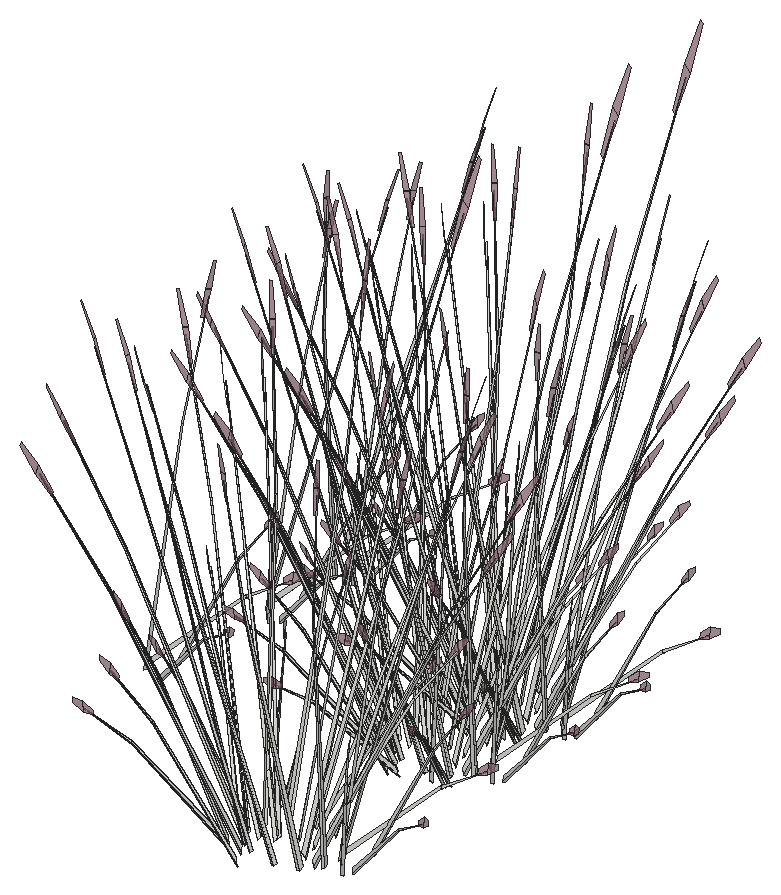
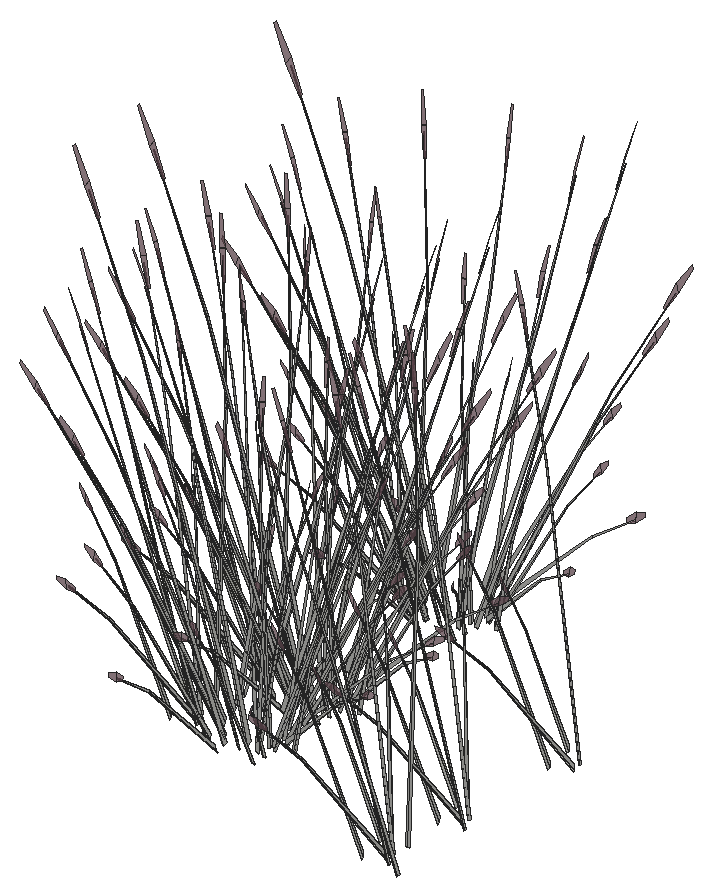
# SketchUp Ruby script. Lengths in inches.
U = 1.inch
M = Sketchup.active_model
def pt(a) = Geom::Point3d.new(a.map { |v| v * U })
def face(e, loops, mat)
  f = e.add_face(loops[0].map { |a| pt(a) })
  loops[1..].each { |l| e.add_face(l.map { |a| pt(a) }).erase! }
  f.material = f.back_material = mat if mat
  f
end
# faces: each face lists its corners as indices into pts; further lists are holes
def faces(e, pts, list, mat = nil) = list.each { |f| face(e, (f[0].is_a?(Array) ? f : [f]).map { |l| l.map { |i| pts[i] } }, mat) }
# xy, xz, yz: faces in a plane at the given z, y or x. An outline is a flat list of corners, or four numbers for a rectangle; further outlines are holes
def ring(l) = l.size == 4 ? [[l[0], l[1]], [l[2], l[1]], [l[2], l[3]], [l[0], l[3]]] : l.each_slice(2).to_a
def flat(e, list, mat, &to3) = list.each { |f| face(e, (f[0].is_a?(Array) ? f : [f]).map { |l| ring(l).map { |u, v| to3.(u, v) } }, mat) }
def xy(e, z, list, mat = nil) = flat(e, list, mat) { |x, y| [x, y, z] }
def xz(e, y, list, mat = nil) = flat(e, list, mat) { |x, z| [x, y, z] }
def yz(e, x, list, mat = nil) = flat(e, list, mat) { |y, z| [x, y, z] }
def lines(e, pts, list) = list.each { |a, b| e.add_line(pt(pts[a]), pt(pts[b])) }
# prism: a flat outline (further loops are holes) pulled along v
def prism(e, loops, v, mat = nil)
  f = face(e, loops, mat); d = Geom::Vector3d.new(v.map { |x| x * U })
  f.pushpull(f.normal.samedirection?(d) ? d.length : -d.length)
end
def box(e, o, s, mat = nil) = prism(e, [[o, [o[0] + s[0], o[1], o[2]], [o[0] + s[0], o[1] + s[1], o[2]], [o[0], o[1] + s[1], o[2]]]], [0, 0, s[2]], mat)
def at(x, y, z, deg = 0) = Geom::Transformation.translation(pt([x, y, z])) * Geom::Transformation.rotation(ORIGIN, Z_AXIS, deg.degrees)
def axes(o, x, y, z) = Geom::Transformation.new([*x, 0, *y, 0, *z, 0, *pt(o).to_a, 1])
def part(name) = M.definitions.add(name)
# library, detail: a bought-in or finely detailed component or shape, given as its bounding box
def library(name, o, s) = part(name).tap { |d| box(d.entities, o, s) }
def detail(e, o, s) = box(e.add_group.entities, o, s)
def put(e, d, t, mat = nil) = e.add_instance(d, t).tap { |i| i.material = mat if mat }
def group(e, t, mat = nil) = e.add_group.tap { |g| g.transformation = t; g.material = mat if mat }.entities
root = M.entities
M.materials.add("LightPink_Translucent").color = [144, 107, 117]
M.materials["LightPink_Translucent"].alpha = 0.75
c1 = part("blade")
p = [[2.15,0.21,22],[0,0.17,0],[0.09,0.45,0],[2.18,0.31,22],[2.29,0.31,22],[0.38,0.45,0],
  [2.48,0.24,33],[2.49,0.24,33],[2.48,0.22,33]]
faces(c1.entities,p,[[0,1,2,3],[4,5,2,3],[6,3,4,7],[8,0,3,6]])
c2 = part("seeds")
p = [[0.3,-0.1,1.38],[-0.01,-0.03,1.59],[-0.01,-0.03,0.03],[0.14,-0.07,-0.07],[0.29,-0.03,3],[0.15,0.01,3.11]]
faces(c2.entities,p,[[0,1,2,3],[1,0,4,5]],"LightPink_Translucent")
c3 = part("blade with seeds")
put(c3.entities,c1,at(0,0,0))
put(c3.entities,c2,axes([2.4,0.25,30.99],[1.5799,-0.05474,1.17369],[-0.12525,1.92788,0.29478],[-0.07173,-0.02425,1.56792]))
put(root,c3,axes([679.98,333.62,514.18],[-0.32734,-0.51701,-0.10093],[0.58097,-0.25407,-0.56021],[0.24483,-0.06821,0.85122]))
put(root,c3,axes([679.89,351.33,514.18],[0.38768,-0.48872,-0.10093],[0.56143,0.28156,-0.56021],[0.19516,0.13808,0.85122]))
put(root,c3,axes([681.9,348.4,514.18],[-0.60181,-0.31483,-0.10093],[0.34671,-0.45593,-0.56021],[0.17003,-0.15849,0.85122]))
put(root,c3,axes([679.82,334.35,513.91],[0.13956,-0.00966,1.45204],[0.38281,-0.44358,-0.22964],[0.24825,0.05855,0.11645]))
put(root,c3,axes([682.43,341.93,513.91],[-0.08498,-0.00434,1.47228],[-0.35287,-0.46464,-0.13912],[0.14171,-0.15278,0.26054]))
put(root,c3,axes([680.24,344.37,514.18],[0.03484,-0.58066,-0.10093],[0.65957,0.01587,-0.56021],[0.25402,0.04034,0.85122]))
put(root,c3,axes([680.97,343.3,514.18],[-0.32734,-0.51701,-0.10093],[0.58097,-0.25407,-0.56021],[0.24483,-0.06821,0.85122]))
put(root,c3,axes([681.28,335.16,513.91],[-0.05883,-0.04999,1.47228],[0.12868,-0.53581,-0.13912],[0.23172,-0.03423,0.26054]))
put(root,c3,axes([680.81,344.02,513.91],[0.13956,-0.00966,1.45204],[0.38281,-0.44358,-0.22964],[0.24825,0.05855,0.11645]))
put(root,c3,axes([683.38,348.26,513.91],[-0.08498,-0.00434,1.47228],[-0.35287,-0.46464,-0.13912],[0.14171,-0.15278,0.26054]))
put(root,c3,axes([681.76,332.81,513.91],[0.09028,-0.08697,1.45204],[-0.11555,-0.53348,-0.22964],[0.22652,-0.10115,0.11645]))
put(root,c3,axes([681.1875,350.7,514.18],[0.03484,-0.58066,-0.10093],[0.65957,0.01587,-0.56021],[0.25402,0.04034,0.85122]))
put(root,c3,axes([681.92,349.63,514.18],[-0.32734,-0.51701,-0.10093],[0.58097,-0.25407,-0.56021],[0.24483,-0.06821,0.85122]))
put(root,c3,axes([682.27,344.83,513.91],[-0.05883,-0.04999,1.47228],[0.12868,-0.53581,-0.13912],[0.23172,-0.03423,0.26054]))
put(root,c3,axes([681.76,350.35,513.91],[0.13956,-0.00966,1.45204],[0.38281,-0.44358,-0.22964],[0.24825,0.05855,0.11645]))
put(root,c3,axes([682.75,342.49,513.91],[0.09028,-0.08697,1.45204],[-0.11555,-0.53348,-0.22964],[0.22652,-0.10115,0.11645]))
put(root,c3,axes([683.22,351.16,513.91],[-0.05883,-0.04999,1.47228],[0.12868,-0.53581,-0.13912],[0.23172,-0.03423,0.26054]))
put(root,c3,axes([683.7,348.82,513.91],[0.09028,-0.08697,1.45204],[-0.11555,-0.53348,-0.22964],[0.22652,-0.10115,0.11645]))
put(root,c3,axes([696.37,321.97,513.22],[0.26985,-0.01293,1.42242],[-0.17902,0.56047,0.11501],[-0.38456,-0.03467,0.60807]))
put(root,c3,axes([696.37,335.47,513.22],[0.26985,-0.01293,1.42242],[-0.17902,0.56047,0.11501],[-0.38456,-0.03467,0.60807]))
put(root,c3,axes([696.37,341.87,513.22],[0.26985,-0.01293,1.42242],[-0.17902,0.56047,0.11501],[-0.38456,-0.03467,0.60807]))
put(root,c3,axes([696.48,322.95,513.22],[0.22574,-0.12077,1.42242],[0.19004,0.55807,0.11501],[-0.35439,0.12613,0.60807]))
put(root,c3,axes([696.48,336.45,513.22],[0.22574,-0.12077,1.42242],[0.19004,0.55807,0.11501],[-0.35439,0.12613,0.60807]))
put(root,c3,axes([696.48,342.85,513.22],[0.22574,-0.12077,1.42242],[0.19004,0.55807,0.11501],[-0.35439,0.12613,0.60807]))
put(root,c3,axes([695.79,322.76,513.91],[-0.10624,0.07413,1.45204],[0.00904,0.54162,-0.22964],[-0.24352,0.07044,0.11645]))
put(root,c3,axes([695.79,336.26,513.91],[-0.10624,0.07413,1.45204],[0.00904,0.54162,-0.22964],[-0.24352,0.07044,0.11645]))
put(root,c3,axes([695.79,342.66,513.91],[-0.10624,0.07413,1.45204],[0.00904,0.54162,-0.22964],[-0.24352,0.07044,0.11645]))
put(root,c3,axes([696.875,321.07,513.22],[0.24166,0.09837,1.42242],[-0.50011,0.41269,0.11501],[-0.3117,-0.18617,0.60807]))
put(root,c3,axes([696.875,334.57,513.22],[0.24166,0.09837,1.42242],[-0.50011,0.41269,0.11501],[-0.3117,-0.18617,0.60807]))
put(root,c3,axes([696.875,340.97,513.22],[0.24166,0.09837,1.42242],[-0.50011,0.41269,0.11501],[-0.3117,-0.18617,0.60807]))
put(root,c3,axes([694.61,323.31,513.91],[0.08303,0.01531,1.47228],[0.25685,0.50448,-0.13912],[-0.16996,0.13241,0.26054]))
put(root,c3,axes([694.61,336.81,513.91],[0.08303,0.01531,1.47228],[0.25685,0.50448,-0.13912],[-0.16996,0.13241,0.26054]))
put(root,c3,axes([694.61,343.21,513.91],[0.08303,0.01531,1.47228],[0.25685,0.50448,-0.13912],[-0.16996,0.13241,0.26054]))
put(root,c3,axes([696.29,320.5,513.91],[0.04823,0.05698,1.47228],[-0.23252,0.51221,-0.13912],[-0.23548,0.00371,0.26054]))
put(root,c3,axes([696.29,334,513.91],[0.04823,0.05698,1.47228],[-0.23252,0.51221,-0.13912],[-0.23548,0.00371,0.26054]))
put(root,c3,axes([696.29,340.4,513.91],[0.04823,0.05698,1.47228],[-0.23252,0.51221,-0.13912],[-0.23548,0.00371,0.26054]))
put(root,c3,axes([696.83,320.16,513.91],[-0.13998,-0.00403,1.45204],[-0.44565,0.40302,-0.22964],[-0.23779,-0.08235,0.11645]))
put(root,c3,axes([696.83,333.66,513.91],[-0.13998,-0.00403,1.45204],[-0.44565,0.40302,-0.22964],[-0.23779,-0.08235,0.11645]))
put(root,c3,axes([696.83,340.0625,513.91],[-0.13998,-0.00403,1.45204],[-0.44565,0.40302,-0.22964],[-0.23779,-0.08235,0.11645]))
put(root,c3,axes([696.47,322.24,514.18],[0.32734,0.51701,-0.10093],[-0.58097,0.25407,-0.56021],[-0.24483,0.06821,0.85122]))
put(root,c3,axes([696.47,335.74,514.18],[0.32734,0.51701,-0.10093],[-0.58097,0.25407,-0.56021],[-0.24483,0.06821,0.85122]))
put(root,c3,axes([696.47,342.14,514.18],[0.32734,0.51701,-0.10093],[-0.58097,0.25407,-0.56021],[-0.24483,0.06821,0.85122]))
put(root,c3,axes([697.21,321.17,514.18],[-0.03484,0.58066,-0.10093],[-0.65957,-0.01587,-0.56021],[-0.25402,-0.04034,0.85122]))
put(root,c3,axes([697.21,334.67,514.18],[-0.03484,0.58066,-0.10093],[-0.65957,-0.01587,-0.56021],[-0.25402,-0.04034,0.85122]))
put(root,c3,axes([697.21,341.07,514.18],[-0.03484,0.58066,-0.10093],[-0.65957,-0.01587,-0.56021],[-0.25402,-0.04034,0.85122]))
put(root,c3,axes([697.31,323.33,513.22],[0.1625,-0.17544,1.42242],[0.41029,0.47354,0.11501],[-0.28141,0.21565,0.60807]))
put(root,c3,axes([697.31,336.83,513.22],[0.1625,-0.17544,1.42242],[0.41029,0.47354,0.11501],[-0.28141,0.21565,0.60807]))
put(root,c3,axes([697.31,343.23,513.22],[0.1625,-0.17544,1.42242],[0.41029,0.47354,0.11501],[-0.28141,0.21565,0.60807]))
put(root,c3,axes([697.18,323.76,513.22],[0.12114,-0.19625,1.42242],[0.50818,0.40613,0.11501],[-0.22925,0.25313,0.60807]))
put(root,c3,axes([697.18,337.26,513.22],[0.12114,-0.19625,1.42242],[0.50818,0.40613,0.11501],[-0.22925,0.25313,0.60807]))
put(root,c3,axes([697.18,343.66,513.22],[0.12114,-0.19625,1.42242],[0.50818,0.40613,0.11501],[-0.22925,0.25313,0.60807]))
put(root,c3,axes([695.81,324.78,513.91],[-0.01617,0.11299,1.45204],[0.45894,0.39307,-0.22964],[-0.12015,0.18588,0.11645]))
put(root,c3,axes([695.81,338.28,513.91],[-0.01617,0.11299,1.45204],[0.45894,0.39307,-0.22964],[-0.12015,0.18588,0.11645]))
put(root,c3,axes([695.81,344.68,513.91],[-0.01617,0.11299,1.45204],[0.45894,0.39307,-0.22964],[-0.12015,0.18588,0.11645]))
put(root,c3,axes([698.49,320.32,514.51],[-0.4342,0.54737,-0.11304],[-0.6288,-0.31535,-0.62743],[-0.21858,-0.15465,0.95337]))
put(root,c3,axes([698.49,333.82,514.51],[-0.4342,0.54737,-0.11304],[-0.6288,-0.31535,-0.62743],[-0.21858,-0.15465,0.95337]))
put(root,c3,axes([698.49,340.22,514.51],[-0.4342,0.54737,-0.11304],[-0.6288,-0.31535,-0.62743],[-0.21858,-0.15465,0.95337]))
put(root,c3,axes([696.5,323.47,514.18],[0.60181,0.31483,-0.10093],[-0.34671,0.45593,-0.56021],[-0.17003,0.15849,0.85122]))
put(root,c3,axes([696.5,336.97,514.18],[0.60181,0.31483,-0.10093],[-0.34671,0.45593,-0.56021],[-0.17003,0.15849,0.85122]))
put(root,c3,axes([696.5,343.37,514.18],[0.60181,0.31483,-0.10093],[-0.34671,0.45593,-0.56021],[-0.17003,0.15849,0.85122]))
put(root,c3,axes([698.33,319.02,513.91],[-0.01214,0.06844,1.47228],[-0.59861,0.24837,-0.13912],[-0.17615,-0.12696,0.26054]))
put(root,c3,axes([698.33,332.52,513.91],[-0.01214,0.06844,1.47228],[-0.59861,0.24837,-0.13912],[-0.17615,-0.12696,0.26054]))
put(root,c3,axes([698.33,338.92,513.91],[-0.01214,0.06844,1.47228],[-0.59861,0.24837,-0.13912],[-0.17615,-0.12696,0.26054]))
put(root,c3,axes([697.87,334,513.22],[0.14872,0.18332,1.42242],[-0.6872,0.15433,0.11501],[-0.15531,-0.28779,0.60807]))
put(root,c3,axes([697.87,340.4,513.22],[0.14872,0.18332,1.42242],[-0.6872,0.15433,0.11501],[-0.15531,-0.28779,0.60807]))
put(root,c3,axes([695.75,325.9375,513.91],[0.07381,-0.03447,1.47228],[0.61004,0.22929,-0.13912],[-0.01434,0.19091,0.26054]))
put(root,c3,axes([695.75,339.4375,513.91],[0.07381,-0.03447,1.47228],[0.61004,0.22929,-0.13912],[-0.01434,0.19091,0.26054]))
put(root,c3,axes([695.75,345.84,513.91],[0.07381,-0.03447,1.47228],[0.61004,0.22929,-0.13912],[-0.01434,0.19091,0.26054]))
put(root,c3,axes([699.01,332.78,513.91],[-0.09951,-0.08005,1.45204],[-0.66407,0.05075,-0.22964],[-0.10598,-0.19148,0.11645]))
put(root,c3,axes([699.01,339.18,513.91],[-0.09951,-0.08005,1.45204],[-0.66407,0.05075,-0.22964],[-0.10598,-0.19148,0.11645]))
put(root,c3,axes([697.27,324.52,514.48],[0.71502,0.02829,-0.11203],[-0.01954,0.53563,-0.62183],[-0.04967,0.20629,0.94486]))
put(root,c3,axes([697.27,338.02,514.48],[0.71502,0.02829,-0.11203],[-0.01954,0.53563,-0.62183],[-0.04967,0.20629,0.94486]))
put(root,c3,axes([697.27,344.42,514.48],[0.71502,0.02829,-0.11203],[-0.01954,0.53563,-0.62183],[-0.04967,0.20629,0.94486]))
put(root,c3,axes([700.02,320.52,514.18],[-0.63664,0.26583,-0.10093],[-0.31286,-0.47181,-0.56021],[-0.084,-0.19882,0.85122]))
put(root,c3,axes([700.02,334.02,514.18],[-0.63664,0.26583,-0.10093],[-0.31286,-0.47181,-0.56021],[-0.084,-0.19882,0.85122]))
put(root,c3,axes([700.02,340.42,514.18],[-0.63664,0.26583,-0.10093],[-0.31286,-0.47181,-0.56021],[-0.084,-0.19882,0.85122]))
put(root,c3,axes([698.29,324.18,513.22],[-0.01592,-0.21915,1.42242],[0.69015,0.14538,0.11501],[-0.04269,0.3123,0.60807]))
put(root,c3,axes([698.29,337.68,513.22],[-0.01592,-0.21915,1.42242],[0.69015,0.14538,0.11501],[-0.04269,0.3123,0.60807]))
put(root,c3,axes([698.29,344.08,513.22],[-0.01592,-0.21915,1.42242],[0.69015,0.14538,0.11501],[-0.04269,0.3123,0.60807]))
put(root,c3,axes([698.45,326.18,513.91],[0.08247,0.09194,1.45204],[0.66552,0.03612,-0.22964],[0.06692,0.20277,0.11645]))
put(root,c3,axes([698.45,339.68,513.91],[0.08247,0.09194,1.45204],[0.66552,0.03612,-0.22964],[0.06692,0.20277,0.11645]))
put(root,c3,axes([698.45,346.08,513.91],[0.08247,0.09194,1.45204],[0.66552,0.03612,-0.22964],[0.06692,0.20277,0.11645]))
put(root,c3,axes([698.6,325.12,514.18],[0.63664,-0.26583,-0.10093],[0.31286,0.47181,-0.56021],[0.084,0.19882,0.85122]))
put(root,c3,axes([698.6,338.62,514.18],[0.63664,-0.26583,-0.10093],[0.31286,0.47181,-0.56021],[0.084,0.19882,0.85122]))
put(root,c3,axes([698.6,345.02,514.18],[0.63664,-0.26583,-0.10093],[0.31286,0.47181,-0.56021],[0.084,0.19882,0.85122]))
put(root,c3,axes([701.85,333.35,513.91],[-0.06607,0.04361,1.47228],[-0.64734,-0.14714,-0.13912],[-0.02343,-0.19032,0.26054]))
put(root,c3,axes([701.85,339.75,513.91],[-0.06607,0.04361,1.47228],[-0.64734,-0.14714,-0.13912],[-0.02343,-0.19032,0.26054]))
put(root,c3,axes([701.34,321.11,514.18],[-0.71502,-0.02829,-0.10093],[0.01954,-0.53563,-0.56021],[0.04967,-0.20629,0.85122]))
put(root,c3,axes([701.34,334.61,514.18],[-0.71502,-0.02829,-0.10093],[0.01954,-0.53563,-0.56021],[0.04967,-0.20629,0.85122]))
put(root,c3,axes([701.34,341.01,514.18],[-0.71502,-0.02829,-0.10093],[0.01954,-0.53563,-0.56021],[0.04967,-0.20629,0.85122]))
put(root,c3,axes([699.51,324.09,513.22],[-0.14872,-0.18332,1.42242],[0.6872,-0.15433,0.11501],[0.15531,0.28779,0.60807]))
put(root,c3,axes([699.51,337.59,513.22],[-0.14872,-0.18332,1.42242],[0.6872,-0.15433,0.11501],[0.15531,0.28779,0.60807]))
put(root,c3,axes([699.51,343.99,513.22],[-0.14872,-0.18332,1.42242],[0.6872,-0.15433,0.11501],[0.15531,0.28779,0.60807]))
put(root,c3,axes([700.55,322.22,513.71],[-0.56218,-0.29666,1.14775],[0.59361,-0.46189,0.49522],[0.18138,0.27836,1.10941]))
put(root,c3,axes([700.55,335.72,513.71],[-0.56218,-0.29666,1.14775],[0.59361,-0.46189,0.49522],[0.18138,0.27836,1.10941]))
put(root,c3,axes([700.55,342.12,513.71],[-0.56218,-0.29666,1.14775],[0.59361,-0.46189,0.49522],[0.18138,0.27836,1.10941]))
put(root,c3,axes([699.6,325.51,513.91],[0.00193,-0.06913,1.47228],[0.55753,-0.30498,-0.13912],[0.19366,0.10886,0.26054]))
put(root,c3,axes([699.6,339.01,513.91],[0.00193,-0.06913,1.47228],[0.55753,-0.30498,-0.13912],[0.19366,0.10886,0.26054]))
put(root,c3,axes([699.6,345.41,513.91],[0.00193,-0.06913,1.47228],[0.55753,-0.30498,-0.13912],[0.19366,0.10886,0.26054]))
put(root,c3,axes([701.99,333.76,513.91],[-0.00628,-0.11364,1.45204],[-0.53042,-0.32843,-0.22964],[0.08201,-0.19909,0.11645]))
put(root,c3,axes([701.99,340.16,513.91],[-0.00628,-0.11364,1.45204],[-0.53042,-0.32843,-0.22964],[0.08201,-0.19909,0.11645]))
put(root,c3,axes([700.19,334.32,513.22],[-0.12114,0.19625,1.42242],[-0.50818,-0.40613,0.11501],[0.22925,-0.25313,0.60807]))
put(root,c3,axes([700.19,340.72,513.22],[-0.12114,0.19625,1.42242],[-0.50818,-0.40613,0.11501],[0.22925,-0.25313,0.60807]))
put(root,c3,axes([700.11,325.1,514.18],[0.38768,-0.48872,-0.10093],[0.56143,0.28156,-0.56021],[0.19516,0.13808,0.85122]))
put(root,c3,axes([700.11,338.6,514.18],[0.38768,-0.48872,-0.10093],[0.56143,0.28156,-0.56021],[0.19516,0.13808,0.85122]))
put(root,c3,axes([700.11,345,514.18],[0.38768,-0.48872,-0.10093],[0.56143,0.28156,-0.56021],[0.19516,0.13808,0.85122]))
put(root,c3,axes([702.12,322.17,514.18],[-0.60181,-0.31483,-0.10093],[0.34671,-0.45593,-0.56021],[0.17003,-0.15849,0.85122]))
put(root,c3,axes([702.12,335.67,514.18],[-0.60181,-0.31483,-0.10093],[0.34671,-0.45593,-0.56021],[0.17003,-0.15849,0.85122]))
put(root,c3,axes([702.12,342.07,514.18],[-0.60181,-0.31483,-0.10093],[0.34671,-0.45593,-0.56021],[0.17003,-0.15849,0.85122]))
put(root,c3,axes([700.5,323.51,513.22],[-0.24166,-0.09837,1.42242],[0.50011,-0.41269,0.11501],[0.3117,0.18617,0.60807]))
put(root,c3,axes([700.5,337.01,513.22],[-0.24166,-0.09837,1.42242],[0.50011,-0.41269,0.11501],[0.3117,0.18617,0.60807]))
put(root,c3,axes([700.5,343.41,513.22],[-0.24166,-0.09837,1.42242],[0.50011,-0.41269,0.11501],[0.3117,0.18617,0.60807]))
put(root,c3,axes([703.6,322.03,513.91],[-0.08498,-0.00434,1.47228],[-0.35287,-0.46464,-0.13912],[0.14171,-0.15278,0.26054]))
put(root,c3,axes([703.6,335.53,513.91],[-0.08498,-0.00434,1.47228],[-0.35287,-0.46464,-0.13912],[0.14171,-0.15278,0.26054]))
put(root,c3,axes([703.6,341.93,513.91],[-0.08498,-0.00434,1.47228],[-0.35287,-0.46464,-0.13912],[0.14171,-0.15278,0.26054]))
put(root,c3,axes([701.41,324.47,514.18],[0.03484,-0.58066,-0.10093],[0.65957,0.01587,-0.56021],[0.25402,0.04034,0.85122]))
put(root,c3,axes([701.41,337.97,514.18],[0.03484,-0.58066,-0.10093],[0.65957,0.01587,-0.56021],[0.25402,0.04034,0.85122]))
put(root,c3,axes([701.41,344.37,514.18],[0.03484,-0.58066,-0.10093],[0.65957,0.01587,-0.56021],[0.25402,0.04034,0.85122]))
put(root,c3,axes([702.14,323.4,514.18],[-0.32734,-0.51701,-0.10093],[0.58097,-0.25407,-0.56021],[0.24483,-0.06821,0.85122]))
put(root,c3,axes([702.14,336.9,514.18],[-0.32734,-0.51701,-0.10093],[0.58097,-0.25407,-0.56021],[0.24483,-0.06821,0.85122]))
put(root,c3,axes([702.14,343.3,514.18],[-0.32734,-0.51701,-0.10093],[0.58097,-0.25407,-0.56021],[0.24483,-0.06821,0.85122]))
put(root,c3,axes([701.98,324.12,513.91],[0.13956,-0.00966,1.45204],[0.38281,-0.44358,-0.22964],[0.24825,0.05855,0.11645]))
put(root,c3,axes([701.98,337.62,513.91],[0.13956,-0.00966,1.45204],[0.38281,-0.44358,-0.22964],[0.24825,0.05855,0.11645]))
put(root,c3,axes([701.98,344.02,513.91],[0.13956,-0.00966,1.45204],[0.38281,-0.44358,-0.22964],[0.24825,0.05855,0.11645]))
put(root,c3,axes([703.44,324.93,513.91],[-0.05883,-0.04999,1.47228],[0.12868,-0.53581,-0.13912],[0.23172,-0.03423,0.26054]))
put(root,c3,axes([703.44,338.43,513.91],[-0.05883,-0.04999,1.47228],[0.12868,-0.53581,-0.13912],[0.23172,-0.03423,0.26054]))
put(root,c3,axes([703.44,344.83,513.91],[-0.05883,-0.04999,1.47228],[0.12868,-0.53581,-0.13912],[0.23172,-0.03423,0.26054]))
put(root,c3,axes([701.01,322.61,513.22],[-0.26985,0.01293,1.42242],[0.17902,-0.56047,0.11501],[0.38456,0.03467,0.60807]))
put(root,c3,axes([701.01,336.11,513.22],[-0.26985,0.01293,1.42242],[0.17902,-0.56047,0.11501],[0.38456,0.03467,0.60807]))
put(root,c3,axes([701.01,342.51,513.22],[-0.26985,0.01293,1.42242],[0.17902,-0.56047,0.11501],[0.38456,0.03467,0.60807]))
put(root,c3,axes([703.92,322.59,513.91],[0.09028,-0.08697,1.45204],[-0.11555,-0.53348,-0.22964],[0.22652,-0.10115,0.11645]))
put(root,c3,axes([703.92,336.09,513.91],[0.09028,-0.08697,1.45204],[-0.11555,-0.53348,-0.22964],[0.22652,-0.10115,0.11645]))
put(root,c3,axes([703.92,342.49,513.91],[0.09028,-0.08697,1.45204],[-0.11555,-0.53348,-0.22964],[0.22652,-0.10115,0.11645]))
